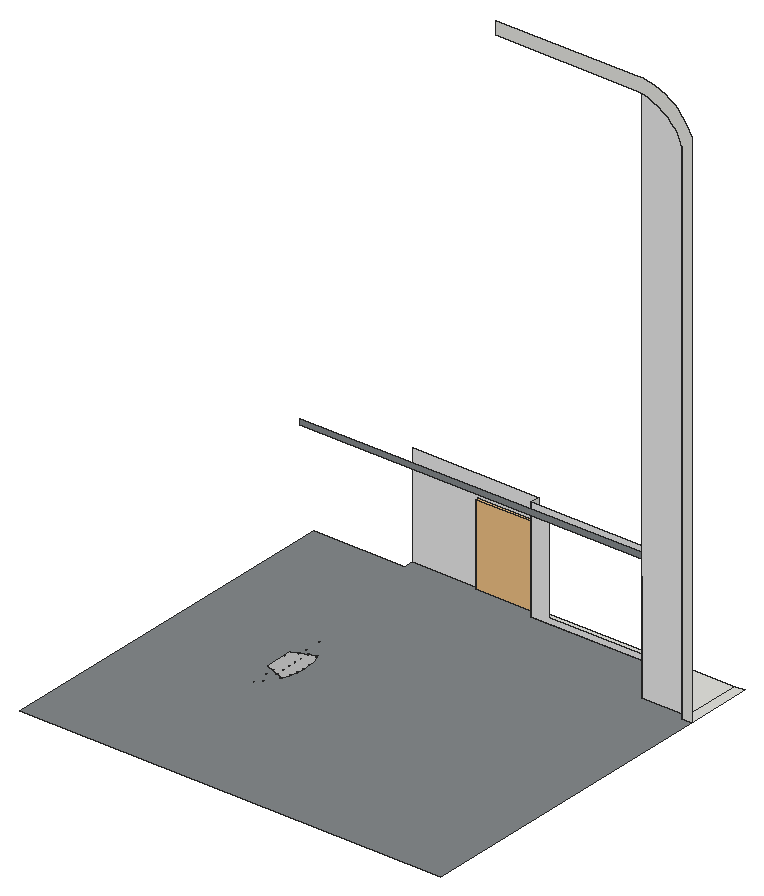
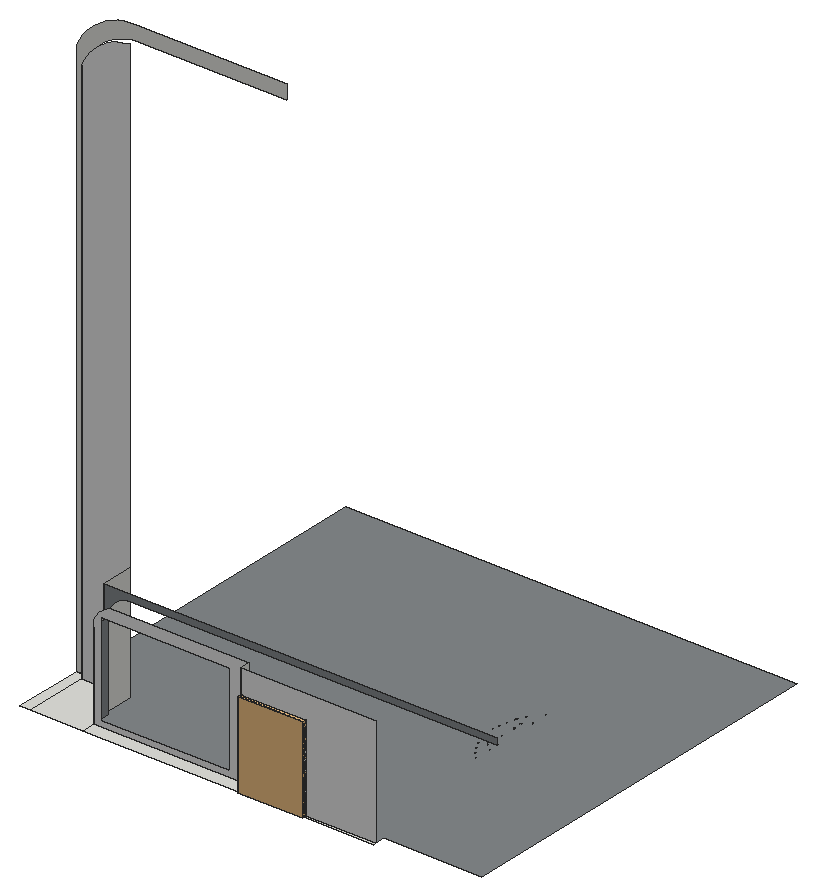
# SketchUp Ruby script. Lengths in inches.
U = 1.inch
M = Sketchup.active_model
def pt(a) = Geom::Point3d.new(a.map { |v| v * U })
def face(e, loops, mat)
  f = e.add_face(loops[0].map { |a| pt(a) })
  loops[1..].each { |l| e.add_face(l.map { |a| pt(a) }).erase! }
  f.material = f.back_material = mat if mat
  f
end
# faces: each face lists its corners as indices into pts; further lists are holes
def faces(e, pts, list, mat = nil) = list.each { |f| face(e, (f[0].is_a?(Array) ? f : [f]).map { |l| l.map { |i| pts[i] } }, mat) }
# xy, xz, yz: faces in a plane at the given z, y or x. An outline is a flat list of corners, or four numbers for a rectangle; further outlines are holes
def ring(l) = l.size == 4 ? [[l[0], l[1]], [l[2], l[1]], [l[2], l[3]], [l[0], l[3]]] : l.each_slice(2).to_a
def flat(e, list, mat, &to3) = list.each { |f| face(e, (f[0].is_a?(Array) ? f : [f]).map { |l| ring(l).map { |u, v| to3.(u, v) } }, mat) }
def xy(e, z, list, mat = nil) = flat(e, list, mat) { |x, y| [x, y, z] }
def xz(e, y, list, mat = nil) = flat(e, list, mat) { |x, z| [x, y, z] }
def yz(e, x, list, mat = nil) = flat(e, list, mat) { |y, z| [x, y, z] }
def lines(e, pts, list) = list.each { |a, b| e.add_line(pt(pts[a]), pt(pts[b])) }
# prism: a flat outline (further loops are holes) pulled along v
def prism(e, loops, v, mat = nil)
  f = face(e, loops, mat); d = Geom::Vector3d.new(v.map { |x| x * U })
  f.pushpull(f.normal.samedirection?(d) ? d.length : -d.length)
end
def box(e, o, s, mat = nil) = prism(e, [[o, [o[0] + s[0], o[1], o[2]], [o[0] + s[0], o[1] + s[1], o[2]], [o[0], o[1] + s[1], o[2]]]], [0, 0, s[2]], mat)
def at(x, y, z, deg = 0) = Geom::Transformation.translation(pt([x, y, z])) * Geom::Transformation.rotation(ORIGIN, Z_AXIS, deg.degrees)
def axes(o, x, y, z) = Geom::Transformation.new([*x, 0, *y, 0, *z, 0, *pt(o).to_a, 1])
def part(name) = M.definitions.add(name)
# library, detail: a bought-in or finely detailed component or shape, given as its bounding box
def library(name, o, s) = part(name).tap { |d| box(d.entities, o, s) }
def detail(e, o, s) = box(e.add_group.entities, o, s)
def put(e, d, t, mat = nil) = e.add_instance(d, t).tap { |i| i.material = mat if mat }
def group(e, t, mat = nil) = e.add_group.tap { |g| g.transformation = t; g.material = mat if mat }.entities
root = M.entities
M.materials.add("[Blacktop Old 01]").color = [132, 136, 139]
M.materials.add("[Metal_Steel_Textured_White]").color = [191, 191, 191]
M.materials.add("[Polished Concrete Old]").color = [229, 229, 229]
c1 = library("Glazed door",[-33.63,86.05,37.23],[27.33,3.12,36.46])
xy(root,3.625,[[303.95,218.965,308.325,249.09],[283.369,221.902,303.95,221.902,303.95,249.09,281.798,249.09,281.798,235.715,283.369,235.715],[215.602,243.402,281.798,249.09],[158.149,247.965,187.79,249.09]])
xy(root,3.625,[[116.615,76.29,308.325,76.29,308.325,218.965,303.95,218.965,303.95,221.902,283.369,221.902,283.369,235.715,281.798,235.715,281.798,243.402,215.602,243.402,215.602,249.09,187.79,249.09,187.79,247.965,158.149,247.965,158.149,243.402,116.615,243.402]],"[Blacktop Old 01]")
xy(root,3.625,[[[168.355,144.804,168.345,144.805,168.337,144.809,168.329,144.815,168.323,144.822,168.32,144.831,168.318,144.84,168.32,144.85,168.323,144.859,168.329,144.866,168.337,144.872,168.345,144.876,168.355,144.877,168.364,144.876,168.373,144.872,168.381,144.866,168.387,144.859,168.39,144.85,168.392,144.84,168.39,144.831,168.387,144.822,168.381,144.815,168.373,144.809,168.364,144.805],[168.355,144.82,168.36,144.821,168.365,144.823,168.369,144.826,168.372,144.83,168.374,144.835,168.375,144.84,168.374,144.846,168.372,144.85,168.369,144.854,168.365,144.858,168.36,144.86,168.35,144.86,168.345,144.858,168.341,144.854,168.338,144.85,168.336,144.846,168.335,144.84,168.336,144.835,168.338,144.83,168.341,144.826,168.345,144.823,168.35,144.821]],[168.355,144.82,168.35,144.821,168.345,144.823,168.341,144.826,168.338,144.83,168.336,144.835,168.335,144.84,168.336,144.846,168.338,144.85,168.341,144.854,168.345,144.858,168.35,144.86,168.36,144.86,168.365,144.858,168.369,144.854,168.372,144.85,168.374,144.846,168.375,144.84,168.374,144.835,168.372,144.83,168.369,144.826,168.365,144.823,168.36,144.821],[[170.535,147.224,170.512,147.227,170.49,147.236,170.472,147.25,170.458,147.269,170.449,147.29,170.446,147.313,170.449,147.336,170.458,147.358,170.472,147.376,170.49,147.39,170.512,147.399,170.535,147.402,170.558,147.399,170.579,147.39,170.597,147.376,170.612,147.358,170.62,147.336,170.624,147.313,170.62,147.29,170.612,147.269,170.597,147.25,170.579,147.236,170.558,147.227],[170.535,147.225,170.557,147.228,170.579,147.237,170.597,147.251,170.611,147.269,170.62,147.29,170.623,147.313,170.62,147.336,170.611,147.357,170.597,147.375,170.579,147.389,170.557,147.398,170.535,147.401,170.512,147.398,170.491,147.389,170.472,147.375,170.458,147.357,170.45,147.336,170.447,147.313,170.45,147.29,170.458,147.269,170.472,147.251,170.491,147.237,170.512,147.228]],[[172.387,149.952,172.364,149.955,172.343,149.964,172.325,149.978,172.311,149.996,172.302,150.017,172.299,150.04,172.302,150.0625,172.311,150.084,172.325,150.102,172.343,150.116,172.364,150.125,172.387,150.128,172.41,150.125,172.431,150.116,172.449,150.102,172.463,150.084,172.472,150.0625,172.475,150.04,172.472,150.017,172.463,149.996,172.449,149.978,172.431,149.964,172.41,149.955],[172.387,150.003,172.396,150.005,172.405,150.008,172.413,150.014,172.418,150.022,172.422,150.03,172.423,150.04,172.422,150.049,172.418,150.058,172.413,150.066,172.405,150.072,172.396,150.075,172.387,150.077,172.377,150.075,172.368,150.072,172.361,150.066,172.355,150.058,172.351,150.049,172.35,150.04,172.351,150.03,172.355,150.022,172.361,150.014,172.368,150.008,172.377,150.005]],[[168.197,151.934,168.174,151.937,168.153,151.946,168.135,151.96,168.121,151.978,168.112,151.999,168.109,152.022,168.112,152.045,168.121,152.066,168.135,152.084,168.153,152.098,168.174,152.107,168.197,152.11,168.22,152.107,168.241,152.098,168.259,152.084,168.273,152.066,168.282,152.045,168.285,152.022,168.282,151.999,168.273,151.978,168.259,151.96,168.241,151.946,168.22,151.937],[168.197,151.985,168.206,151.986,168.215,151.99,168.223,151.996,168.228,152.003,168.232,152.012,168.233,152.022,168.232,152.031,168.228,152.04,168.223,152.048,168.215,152.053,168.206,152.057,168.197,152.058,168.187,152.057,168.178,152.053,168.171,152.048,168.165,152.04,168.161,152.031,168.16,152.022,168.161,152.012,168.165,152.003,168.171,151.996,168.178,151.99,168.187,151.986]],
  [168.192,152.002,168.187,152.004,168.179,152.012,168.177,152.017,168.177,152.027,168.179,152.032,168.183,152.036,168.187,152.039,168.192,152.041,168.197,152.042,168.202,152.041,168.207,152.039,168.211,152.036,168.214,152.032,168.216,152.027,168.217,152.022,168.216,152.017,168.214,152.012,168.211,152.008,168.207,152.004,168.202,152.002],[[173.882,152.889,173.859,152.892,173.838,152.901,173.819,152.915,173.805,152.933,173.796,152.955,173.793,152.978,173.796,153.001,173.805,153.022,173.819,153.04,173.838,153.055,173.859,153.063,173.882,153.066,173.905,153.063,173.927,153.055,173.945,153.04,173.959,153.022,173.968,153.001,173.971,152.978,173.968,152.955,173.959,152.933,173.945,152.915,173.927,152.901,173.905,152.892],[173.882,152.89,173.905,152.893,173.926,152.901,173.944,152.915,173.958,152.934,173.967,152.955,173.97,152.978,173.967,153,173.958,153.022,173.944,153.04,173.926,153.054,173.905,153.0625,173.882,153.066,173.859,153.0625,173.838,153.054,173.82,153.04,173.806,153.022,173.797,153,173.794,152.978,173.797,152.955,173.806,152.934,173.82,152.915,173.838,152.901,173.859,152.893]],[[173.882,152.941,173.873,152.942,173.864,152.946,173.856,152.952,173.85,152.959,173.847,152.968,173.846,152.978,173.847,152.987,173.85,152.996,173.856,153.003,173.864,153.009,173.873,153.013,173.882,153.014,173.892,153.013,173.9,153.009,173.908,153.003,173.914,152.996,173.917,152.987,173.919,152.978,173.917,152.968,173.914,152.959,173.908,152.952,173.9,152.946,173.892,152.942],[173.877,152.958,173.887,152.958,173.892,152.96,173.896,152.963,173.899,152.968,173.901,152.972,173.902,152.978,173.901,152.983,173.899,152.988,173.896,152.992,173.892,152.995,173.887,152.997,173.882,152.998,173.877,152.997,173.872,152.995,173.868,152.992,173.865,152.988,173.863,152.983,173.862,152.978,173.863,152.972,173.865,152.968,173.868,152.963,173.872,152.96]],[173.877,152.958,173.872,152.96,173.868,152.963,173.865,152.968,173.863,152.972,173.862,152.978,173.863,152.983,173.865,152.988,173.868,152.992,173.872,152.995,173.877,152.997,173.882,152.998,173.887,152.997,173.892,152.995,173.896,152.992,173.899,152.988,173.901,152.983,173.902,152.978,173.901,152.972,173.899,152.968,173.896,152.963,173.892,152.96,173.887,152.958],[[174.407,153.192,164.789,157.176,164.789,169.578,174.407,173.5625,175.02,171.932,175.526,170.266,175.921,168.57,176.205,166.851,176.375,165.118,176.432,163.377,176.375,161.637,176.205,159.904,175.921,158.185,175.526,156.489,175.02,154.822],[175.826,166.578,175.849,166.581,175.87,166.59,175.889,166.604,175.903,166.623,175.912,166.644,175.915,166.667,175.912,166.69,175.903,166.712,175.889,166.73,175.87,166.744,175.849,166.753,175.826,166.756,175.803,166.753,175.782,166.744,175.763,166.73,175.749,166.712,175.74,166.69,175.737,166.667,175.74,166.644,175.749,166.623,175.763,166.604,175.782,166.59,175.803,166.581],[174.1875,172.951,174.211,172.954,174.232,172.963,174.251,172.977,174.265,172.995,174.274,173.017,174.277,173.04,174.274,173.0625,174.265,173.084,174.251,173.102,174.232,173.117,174.211,173.125,174.1875,173.128,174.165,173.125,174.143,173.117,174.125,173.102,174.111,173.084,174.102,173.0625,174.099,173.04,174.102,173.017,174.111,172.995,174.125,172.977,174.143,172.963,174.165,172.954],[175.208,156.761,175.231,156.764,175.252,156.773,175.27,156.787,175.285,156.805,175.293,156.827,175.296,156.85,175.293,156.873,175.285,156.894,175.27,156.913,175.252,156.927,175.231,156.936,175.208,156.939,175.185,156.936,175.163,156.927,175.145,156.913,175.131,156.894,175.122,156.873,175.119,156.85,175.122,156.827,175.131,156.805,175.145,156.787,175.163,156.773,175.185,156.764],[170.843,161.633,170.866,161.636,170.888,161.645,170.906,161.659,170.92,161.678,170.929,161.699,170.932,161.722,170.929,161.745,170.92,161.766,170.906,161.785,170.888,161.799,170.866,161.808,170.843,161.811,170.82,161.808,170.799,161.799,170.781,161.785,170.766,161.766,170.758,161.745,170.754,161.722,170.758,161.699,170.766,161.678,170.781,161.659,170.799,161.645,170.82,161.636],[165.188,169.223,165.211,169.226,165.232,169.235,165.251,169.249,165.265,169.267,165.274,169.289,165.277,169.312,165.274,169.335,165.265,169.356,165.251,169.375,165.232,169.389,165.211,169.398,165.188,169.401,165.165,169.398,165.143,169.389,165.125,169.375,165.111,169.356,165.102,169.335,165.099,169.312,165.102,169.289,165.111,169.267,165.125,169.249,165.143,169.235,165.165,169.226],[175.826,159.999,175.849,160.002,175.87,160.011,175.889,160.025,175.903,160.043,175.912,160.065,175.915,160.088,175.912,160.111,175.903,160.132,175.889,160.15,175.87,160.165,175.849,160.173,175.826,160.177,175.803,160.173,175.782,160.165,175.763,160.15,175.749,160.132,175.74,160.111,175.737,160.088,175.74,160.065,175.749,160.043,175.763,160.025,175.782,160.011,175.803,160.002],[168.188,156.112,168.211,156.115,168.232,156.124,168.251,156.138,168.265,156.156,168.274,156.177,168.277,156.2,168.274,156.223,168.265,156.245,168.251,156.263,168.232,156.277,168.211,156.286,168.188,156.289,168.165,156.286,168.143,156.277,168.125,156.263,168.111,156.245,168.102,156.223,168.099,156.2,168.102,156.177,168.111,156.156,168.125,156.138,168.143,156.124,168.165,156.115],[175.208,169.816,175.231,169.819,175.252,169.828,175.27,169.842,175.285,169.861,175.293,169.882,175.296,169.905,175.293,169.928,175.285,169.949,175.27,169.968,175.252,169.982,175.231,169.991,175.208,169.994,175.185,169.991,175.163,169.982,175.145,169.968,175.131,169.949,175.122,169.928,175.119,169.905,175.122,169.882,175.131,169.861,175.145,169.842,175.163,169.828,175.185,169.819],[165.188,160.321,165.211,160.324,165.232,160.333,165.251,160.347,165.265,160.366,165.274,160.387,165.277,160.41,165.274,160.433,165.265,160.455,165.251,160.473,165.232,160.487,165.211,160.496,165.188,160.499,165.165,160.496,165.143,160.487,165.125,160.473,165.111,160.455,165.102,160.433,165.099,160.41,165.102,160.387,165.111,160.366,165.125,160.347,165.143,160.333,165.165,160.324],[165.188,163.289,165.211,163.292,165.232,163.3,165.251,163.315,165.265,163.333,165.274,163.354,165.277,163.377,165.274,163.4,165.265,163.422,165.251,163.44,165.232,163.454,165.211,163.463,165.188,163.466,165.165,163.463,165.143,163.454,165.125,163.44,165.111,163.422,165.102,163.4,165.099,163.377,165.102,163.354,165.111,163.333,165.125,163.315,165.143,163.3,165.165,163.292],[170.843,158.322,170.866,158.325,170.888,158.334,170.906,158.348,170.92,158.367,170.929,158.388,170.932,158.411,170.929,158.434,170.92,158.456,170.906,158.474,170.888,158.488,170.866,158.497,170.843,158.5,170.82,158.497,170.799,158.488,170.781,158.474,170.766,158.456,170.758,158.434,170.754,158.411,170.758,158.388,170.766,158.367,170.781,158.348,170.799,158.334,170.82,158.325],[165.188,166.256,165.211,166.259,165.232,166.268,165.251,166.282,165.265,166.3,165.274,166.322,165.277,166.345,165.274,166.368,165.265,166.389,165.251,166.407,165.232,166.422,165.211,166.43,165.188,166.433,165.165,166.43,165.143,166.422,165.125,166.407,165.111,166.389,165.102,166.368,165.099,166.345,165.102,166.322,165.111,166.3,165.125,166.282,165.143,166.268,165.165,166.259],[168.188,170.465,168.211,170.468,168.232,170.477,168.251,170.492,168.265,170.51,168.274,170.531,168.277,170.554,168.274,170.577,168.265,170.599,168.251,170.617,168.232,170.631,168.211,170.64,168.188,170.643,168.165,170.64,168.143,170.631,168.125,170.617,168.111,170.599,168.102,170.577,168.099,170.554,168.102,170.531,168.111,170.51,168.125,170.492,168.143,170.477,168.165,170.468],[174.1875,153.626,174.211,153.629,174.232,153.638,174.251,153.652,174.265,153.671,174.274,153.692,174.277,153.715,174.274,153.738,174.265,153.76,174.251,153.778,174.232,153.792,174.211,153.801,174.1875,153.804,174.165,153.801,174.143,153.792,174.125,153.778,174.111,153.76,174.102,153.738,174.099,153.715,174.102,153.692,174.111,153.671,174.125,153.652,174.143,153.638,174.165,153.629],[165.188,157.354,165.211,157.357,165.232,157.366,165.251,157.38,165.265,157.399,165.274,157.42,165.277,157.443,165.274,157.466,165.265,157.488,165.251,157.506,165.232,157.52,165.211,157.529,165.188,157.532,165.165,157.529,165.143,157.52,165.125,157.506,165.111,157.488,165.102,157.466,165.099,157.443,165.102,157.42,165.111,157.399,165.125,157.38,165.143,157.366,165.165,157.357],[171.188,154.869,171.211,154.872,171.232,154.881,171.251,154.895,171.265,154.913,171.274,154.935,171.277,154.958,171.274,154.981,171.265,155.002,171.251,155.021,171.232,155.035,171.211,155.044,171.188,155.047,171.165,155.044,171.143,155.035,171.125,155.021,171.111,155.002,171.102,154.981,171.099,154.958,171.102,154.935,171.111,154.913,171.125,154.895,171.143,154.881,171.165,154.872],[170.843,168.255,170.866,168.258,170.888,168.267,170.906,168.281,170.92,168.299,170.929,168.321,170.932,168.344,170.929,168.367,170.92,168.388,170.906,168.406,170.888,168.421,170.866,168.429,170.843,168.432,170.82,168.429,170.799,168.421,170.781,168.406,170.766,168.388,170.758,168.367,170.754,168.344,170.758,168.321,170.766,168.299,170.781,168.281,170.799,168.267,170.82,168.258],[171.188,171.708,171.211,171.711,171.232,171.72,171.251,171.734,171.265,171.753,171.274,171.774,171.277,171.797,171.274,171.82,171.265,171.841,171.251,171.86,171.232,171.874,171.211,171.883,171.188,171.886,171.165,171.883,171.143,171.874,171.125,171.86,171.111,171.841,171.102,171.82,171.099,171.797,171.102,171.774,171.111,171.753,171.125,171.734,171.143,171.72,171.165,171.711],[170.843,164.944,170.866,164.947,170.888,164.956,170.906,164.97,170.92,164.988,170.929,165.01,170.932,165.033,170.929,165.056,170.92,165.077,170.906,165.096,170.888,165.11,170.866,165.119,170.843,165.122,170.82,165.119,170.799,165.11,170.781,165.096,170.766,165.077,170.758,165.056,170.754,165.033,170.758,165.01,170.766,164.988,170.781,164.97,170.799,164.956,170.82,164.947],[176.033,163.289,176.056,163.292,176.078,163.3,176.096,163.315,176.11,163.333,176.119,163.354,176.122,163.377,176.119,163.4,176.11,163.422,176.096,163.44,176.078,163.454,176.056,163.463,176.033,163.466,176.01,163.463,175.989,163.454,175.97,163.44,175.956,163.422,175.947,163.4,175.944,163.377,175.947,163.354,175.956,163.333,175.97,163.315,175.989,163.3,176.01,163.292]],
  [174.1875,153.695,174.183,153.696,174.178,153.698,174.174,153.701,174.17,153.705,174.168,153.71,174.168,153.72,174.17,153.725,174.178,153.733,174.183,153.735,174.193,153.735,174.198,153.733,174.202,153.729,174.205,153.725,174.207,153.72,174.208,153.715,174.207,153.71,174.205,153.705,174.202,153.701,174.198,153.698,174.193,153.696],[[170.882,154.184,170.873,154.185,170.864,154.189,170.856,154.194,170.85,154.202,170.847,154.211,170.846,154.22,170.847,154.23,170.85,154.239,170.856,154.246,170.864,154.252,170.873,154.256,170.882,154.257,170.892,154.256,170.9,154.252,170.908,154.246,170.914,154.239,170.918,154.23,170.919,154.22,170.918,154.211,170.914,154.202,170.908,154.194,170.9,154.189,170.892,154.185],[170.882,154.2,170.887,154.201,170.892,154.203,170.896,154.206,170.899,154.21,170.901,154.215,170.902,154.22,170.901,154.225,170.899,154.23,170.896,154.234,170.892,154.237,170.887,154.239,170.882,154.24,170.877,154.239,170.872,154.237,170.868,154.234,170.865,154.23,170.863,154.225,170.862,154.22,170.863,154.215,170.865,154.21,170.868,154.206,170.872,154.203,170.877,154.201]],[170.882,154.2,170.877,154.201,170.872,154.203,170.868,154.206,170.865,154.21,170.863,154.215,170.862,154.22,170.863,154.225,170.865,154.23,170.868,154.234,170.872,154.237,170.877,154.239,170.882,154.24,170.887,154.239,170.892,154.237,170.896,154.234,170.899,154.23,170.901,154.225,170.902,154.22,170.901,154.215,170.899,154.21,170.896,154.206,170.892,154.203,170.887,154.201],[[171.188,154.921,171.178,154.923,171.169,154.926,171.162,154.932,171.156,154.94,171.152,154.948,171.151,154.958,171.152,154.967,171.156,154.976,171.162,154.984,171.169,154.99,171.178,154.993,171.188,154.994,171.197,154.993,171.206,154.99,171.214,154.984,171.219,154.976,171.223,154.967,171.224,154.958,171.223,154.948,171.219,154.94,171.214,154.932,171.206,154.926,171.197,154.923],[171.188,154.938,171.193,154.939,171.198,154.941,171.202,154.944,171.205,154.948,171.207,154.953,171.208,154.958,171.207,154.963,171.205,154.968,171.202,154.972,171.198,154.975,171.193,154.977,171.188,154.978,171.183,154.977,171.178,154.975,171.174,154.972,171.17,154.968,171.168,154.963,171.168,154.953,171.17,154.948,171.174,154.944,171.178,154.941,171.183,154.939]],[171.188,154.938,171.183,154.939,171.178,154.941,171.174,154.944,171.17,154.948,171.168,154.953,171.168,154.963,171.17,154.968,171.174,154.972,171.178,154.975,171.183,154.977,171.188,154.978,171.193,154.977,171.198,154.975,171.202,154.972,171.205,154.968,171.207,154.963,171.208,154.958,171.207,154.953,171.205,154.948,171.202,154.944,171.198,154.941,171.193,154.939],
  [[175.208,156.761,175.185,156.764,175.163,156.773,175.145,156.787,175.131,156.805,175.122,156.827,175.119,156.85,175.122,156.873,175.131,156.894,175.145,156.913,175.163,156.927,175.185,156.936,175.208,156.939,175.231,156.936,175.252,156.927,175.27,156.913,175.285,156.894,175.293,156.873,175.296,156.85,175.293,156.827,175.285,156.805,175.27,156.787,175.252,156.773,175.231,156.764],[175.208,156.762,175.23,156.765,175.252,156.774,175.27,156.788,175.284,156.806,175.292,156.827,175.295,156.85,175.292,156.873,175.284,156.894,175.27,156.912,175.252,156.926,175.23,156.935,175.208,156.938,175.185,156.935,175.164,156.926,175.145,156.912,175.131,156.894,175.123,156.873,175.12,156.85,175.123,156.827,175.131,156.806,175.145,156.788,175.164,156.774,175.185,156.765]],[[175.208,156.813,175.198,156.814,175.189,156.818,175.182,156.824,175.176,156.832,175.172,156.84,175.171,156.85,175.172,156.859,175.176,156.868,175.182,156.876,175.189,156.882,175.198,156.885,175.208,156.886,175.217,156.885,175.226,156.882,175.233,156.876,175.239,156.868,175.243,156.859,175.244,156.85,175.243,156.84,175.239,156.832,175.233,156.824,175.226,156.818,175.217,156.814],[175.208,156.83,175.213,156.831,175.218,156.833,175.222,156.836,175.225,156.84,175.227,156.845,175.227,156.855,175.225,156.86,175.222,156.864,175.218,156.867,175.213,156.869,175.208,156.87,175.202,156.869,175.198,156.867,175.193,156.864,175.19,156.86,175.188,156.855,175.1875,156.85,175.188,156.845,175.19,156.84,175.193,156.836,175.198,156.833,175.202,156.831]],[175.208,156.83,175.202,156.831,175.198,156.833,175.193,156.836,175.19,156.84,175.188,156.845,175.1875,156.85,175.188,156.855,175.19,156.86,175.193,156.864,175.198,156.867,175.202,156.869,175.208,156.87,175.213,156.869,175.218,156.867,175.222,156.864,175.225,156.86,175.227,156.855,175.227,156.845,175.225,156.84,175.222,156.836,175.218,156.833,175.213,156.831],[[170.843,158.322,170.82,158.325,170.799,158.334,170.781,158.348,170.766,158.367,170.758,158.388,170.754,158.411,170.758,158.434,170.766,158.456,170.781,158.474,170.799,158.488,170.82,158.497,170.843,158.5,170.866,158.497,170.888,158.488,170.906,158.474,170.92,158.456,170.929,158.434,170.932,158.411,170.929,158.388,170.92,158.367,170.906,158.348,170.888,158.334,170.866,158.325],[170.843,158.323,170.866,158.326,170.887,158.335,170.906,158.349,170.92,158.367,170.928,158.389,170.931,158.411,170.928,158.434,170.92,158.455,170.906,158.473,170.887,158.487,170.866,158.496,170.843,158.499,170.821,158.496,170.799,158.487,170.781,158.473,170.767,158.455,170.758,158.434,170.755,158.411,170.758,158.389,170.767,158.367,170.781,158.349,170.799,158.335,170.821,158.326]],[[170.843,158.323,170.821,158.326,170.799,158.335,170.781,158.349,170.767,158.367,170.758,158.389,170.755,158.411,170.758,158.434,170.767,158.455,170.781,158.473,170.799,158.487,170.821,158.496,170.843,158.499,170.866,158.496,170.887,158.487,170.906,158.473,170.92,158.455,170.928,158.434,170.931,158.411,170.928,158.389,170.92,158.367,170.906,158.349,170.887,158.335,170.866,158.326],[170.843,158.375,170.853,158.376,170.862,158.38,170.869,158.385,170.875,158.393,170.879,158.402,170.88,158.411,170.879,158.421,170.875,158.43,170.869,158.437,170.862,158.443,170.853,158.447,170.843,158.448,170.834,158.447,170.825,158.443,170.818,158.437,170.812,158.43,170.808,158.421,170.807,158.411,170.808,158.402,170.812,158.393,170.818,158.385,170.825,158.38,170.834,158.376]],
  [170.843,158.391,170.838,158.392,170.833,158.394,170.829,158.397,170.826,158.401,170.824,158.406,170.823,158.411,170.824,158.416,170.826,158.421,170.829,158.425,170.833,158.429,170.838,158.431,170.849,158.431,170.853,158.429,170.858,158.425,170.861,158.421,170.863,158.416,170.863,158.406,170.861,158.401,170.858,158.397,170.853,158.394,170.849,158.392],[[175.826,159.999,175.803,160.002,175.782,160.011,175.763,160.025,175.749,160.043,175.74,160.065,175.737,160.088,175.74,160.111,175.749,160.132,175.763,160.15,175.782,160.165,175.803,160.173,175.826,160.177,175.849,160.173,175.87,160.165,175.889,160.15,175.903,160.132,175.912,160.111,175.915,160.088,175.912,160.065,175.903,160.043,175.889,160.025,175.87,160.011,175.849,160.002],[175.826,160,175.849,160.003,175.87,160.011,175.888,160.025,175.902,160.044,175.911,160.065,175.914,160.088,175.911,160.11,175.902,160.132,175.888,160.15,175.87,160.164,175.849,160.173,175.826,160.176,175.803,160.173,175.782,160.164,175.764,160.15,175.75,160.132,175.741,160.11,175.738,160.088,175.741,160.065,175.75,160.044,175.764,160.025,175.782,160.011,175.803,160.003]],[[175.826,160.051,175.817,160.052,175.808,160.056,175.8,160.062,175.794,160.069,175.791,160.078,175.789,160.088,175.791,160.097,175.794,160.106,175.8,160.113,175.808,160.119,175.817,160.123,175.826,160.124,175.835,160.123,175.844,160.119,175.852,160.113,175.858,160.106,175.861,160.097,175.863,160.088,175.861,160.078,175.858,160.069,175.852,160.062,175.844,160.056,175.835,160.052],[175.821,160.068,175.831,160.068,175.836,160.07,175.84,160.074,175.843,160.078,175.845,160.082,175.846,160.088,175.845,160.093,175.843,160.098,175.84,160.102,175.836,160.105,175.831,160.107,175.826,160.108,175.821,160.107,175.816,160.105,175.812,160.102,175.809,160.098,175.807,160.093,175.806,160.088,175.807,160.082,175.809,160.078,175.812,160.074,175.816,160.07]],[175.821,160.068,175.816,160.07,175.812,160.074,175.809,160.078,175.807,160.082,175.806,160.088,175.807,160.093,175.809,160.098,175.812,160.102,175.816,160.105,175.821,160.107,175.826,160.108,175.831,160.107,175.836,160.105,175.84,160.102,175.843,160.098,175.845,160.093,175.846,160.088,175.845,160.082,175.843,160.078,175.84,160.074,175.836,160.07,175.831,160.068],[[170.843,161.633,170.82,161.636,170.799,161.645,170.781,161.659,170.766,161.678,170.758,161.699,170.754,161.722,170.758,161.745,170.766,161.766,170.781,161.785,170.799,161.799,170.82,161.808,170.843,161.811,170.866,161.808,170.888,161.799,170.906,161.785,170.92,161.766,170.929,161.745,170.932,161.722,170.929,161.699,170.92,161.678,170.906,161.659,170.888,161.645,170.866,161.636],[170.843,161.634,170.866,161.637,170.887,161.646,170.906,161.66,170.92,161.678,170.928,161.699,170.931,161.722,170.928,161.745,170.92,161.766,170.906,161.784,170.887,161.798,170.866,161.807,170.843,161.81,170.821,161.807,170.799,161.798,170.781,161.784,170.767,161.766,170.758,161.745,170.755,161.722,170.758,161.699,170.767,161.678,170.781,161.66,170.799,161.646,170.821,161.637]],
  [[170.843,161.634,170.821,161.637,170.799,161.646,170.781,161.66,170.767,161.678,170.758,161.699,170.755,161.722,170.758,161.745,170.767,161.766,170.781,161.784,170.799,161.798,170.821,161.807,170.843,161.81,170.866,161.807,170.887,161.798,170.906,161.784,170.92,161.766,170.928,161.745,170.931,161.722,170.928,161.699,170.92,161.678,170.906,161.66,170.887,161.646,170.866,161.637],[170.843,161.685,170.853,161.687,170.862,161.69,170.869,161.696,170.875,161.704,170.879,161.713,170.88,161.722,170.879,161.732,170.875,161.74,170.869,161.748,170.862,161.754,170.853,161.757,170.843,161.759,170.834,161.757,170.825,161.754,170.818,161.748,170.812,161.74,170.808,161.732,170.807,161.722,170.808,161.713,170.812,161.704,170.818,161.696,170.825,161.69,170.834,161.687]],[175.944,163.377,175.947,163.4,175.956,163.422,175.97,163.44,175.989,163.454,176.01,163.463,176.033,163.466,176.056,163.463,176.078,163.454,176.096,163.44,176.11,163.422,176.119,163.4,176.122,163.377,176.121,163.377,176.118,163.4,176.109,163.421,176.095,163.44,176.077,163.454,176.056,163.462,176.033,163.465,176.01,163.462,175.989,163.454,175.971,163.44,175.957,163.421,175.948,163.4,175.945,163.377],[[170.843,164.944,170.82,164.947,170.799,164.956,170.781,164.97,170.766,164.988,170.758,165.01,170.754,165.033,170.758,165.056,170.766,165.077,170.781,165.096,170.799,165.11,170.82,165.119,170.843,165.122,170.866,165.119,170.888,165.11,170.906,165.096,170.92,165.077,170.929,165.056,170.932,165.033,170.929,165.01,170.92,164.988,170.906,164.97,170.888,164.956,170.866,164.947],[170.843,164.945,170.866,164.948,170.887,164.957,170.906,164.971,170.92,164.989,170.928,165.01,170.931,165.033,170.928,165.056,170.92,165.077,170.906,165.095,170.887,165.109,170.866,165.118,170.843,165.121,170.821,165.118,170.799,165.109,170.781,165.095,170.767,165.077,170.758,165.056,170.755,165.033,170.758,165.01,170.767,164.989,170.781,164.971,170.799,164.957,170.821,164.948]],[170.843,165.013,170.838,165.014,170.833,165.016,170.829,165.019,170.826,165.023,170.824,165.028,170.823,165.033,170.824,165.038,170.826,165.043,170.829,165.047,170.833,165.05,170.838,165.052,170.843,165.053,170.849,165.052,170.853,165.05,170.858,165.047,170.861,165.043,170.863,165.038,170.863,165.028,170.861,165.023,170.858,165.019,170.853,165.016,170.849,165.014],[[170.843,168.255,170.82,168.258,170.799,168.267,170.781,168.281,170.766,168.299,170.758,168.321,170.754,168.344,170.758,168.367,170.766,168.388,170.781,168.406,170.799,168.421,170.82,168.429,170.843,168.432,170.866,168.429,170.888,168.421,170.906,168.406,170.92,168.388,170.929,168.367,170.932,168.344,170.929,168.321,170.92,168.299,170.906,168.281,170.888,168.267,170.866,168.258],[170.843,168.256,170.866,168.259,170.887,168.267,170.906,168.281,170.92,168.3,170.928,168.321,170.931,168.344,170.928,168.366,170.92,168.388,170.906,168.406,170.887,168.42,170.866,168.429,170.843,168.432,170.821,168.429,170.799,168.42,170.781,168.406,170.767,168.388,170.758,168.366,170.755,168.344,170.758,168.321,170.767,168.3,170.781,168.281,170.799,168.267,170.821,168.259]],
  [[170.843,168.256,170.821,168.259,170.799,168.267,170.781,168.281,170.767,168.3,170.758,168.321,170.755,168.344,170.758,168.366,170.767,168.388,170.781,168.406,170.799,168.42,170.821,168.429,170.843,168.432,170.866,168.429,170.887,168.42,170.906,168.406,170.92,168.388,170.928,168.366,170.931,168.344,170.928,168.321,170.92,168.3,170.906,168.281,170.887,168.267,170.866,168.259],[170.843,168.307,170.853,168.308,170.862,168.312,170.869,168.318,170.875,168.325,170.879,168.334,170.88,168.344,170.879,168.353,170.875,168.362,170.869,168.369,170.862,168.375,170.853,168.379,170.843,168.38,170.834,168.379,170.825,168.375,170.818,168.369,170.812,168.362,170.808,168.353,170.807,168.344,170.808,168.334,170.812,168.325,170.818,168.318,170.825,168.312,170.834,168.308]],[[168.188,170.465,168.165,170.468,168.143,170.477,168.125,170.492,168.111,170.51,168.102,170.531,168.099,170.554,168.102,170.577,168.111,170.599,168.125,170.617,168.143,170.631,168.165,170.64,168.188,170.643,168.211,170.64,168.232,170.631,168.251,170.617,168.265,170.599,168.274,170.577,168.277,170.554,168.274,170.531,168.265,170.51,168.251,170.492,168.232,170.477,168.211,170.468],[168.188,170.466,168.211,170.469,168.232,170.478,168.25,170.492,168.264,170.51,168.273,170.532,168.276,170.554,168.273,170.577,168.264,170.598,168.25,170.617,168.232,170.631,168.211,170.639,168.188,170.642,168.165,170.639,168.144,170.631,168.126,170.617,168.112,170.598,168.103,170.577,168.1,170.554,168.103,170.532,168.112,170.51,168.126,170.492,168.144,170.478,168.165,170.469]],[[168.188,170.518,168.178,170.519,168.169,170.523,168.162,170.528,168.156,170.536,168.152,170.545,168.151,170.554,168.152,170.564,168.156,170.573,168.162,170.58,168.169,170.586,168.178,170.59,168.188,170.591,168.197,170.59,168.206,170.586,168.214,170.58,168.219,170.573,168.223,170.564,168.224,170.554,168.223,170.545,168.219,170.536,168.214,170.528,168.206,170.523,168.197,170.519],[168.188,170.534,168.193,170.535,168.198,170.537,168.202,170.54,168.205,170.544,168.207,170.549,168.208,170.554,168.207,170.56,168.205,170.564,168.202,170.568,168.198,170.572,168.193,170.574,168.183,170.574,168.178,170.572,168.17,170.564,168.168,170.56,168.168,170.549,168.17,170.544,168.174,170.54,168.178,170.537,168.183,170.535]],[168.188,170.534,168.183,170.535,168.178,170.537,168.174,170.54,168.17,170.544,168.168,170.549,168.168,170.56,168.17,170.564,168.178,170.572,168.183,170.574,168.193,170.574,168.198,170.572,168.202,170.568,168.205,170.564,168.207,170.56,168.208,170.554,168.207,170.549,168.205,170.544,168.202,170.54,168.198,170.537,168.193,170.535],[[167.882,171.203,167.859,171.206,167.838,171.215,167.819,171.229,167.805,171.248,167.796,171.269,167.793,171.292,167.796,171.315,167.805,171.336,167.819,171.355,167.838,171.369,167.859,171.378,167.882,171.381,167.905,171.378,167.927,171.369,167.945,171.355,167.959,171.336,167.968,171.315,167.971,171.292,167.968,171.269,167.959,171.248,167.945,171.229,167.927,171.215,167.905,171.206],[167.882,171.204,167.905,171.207,167.926,171.216,167.944,171.23,167.958,171.248,167.967,171.269,167.97,171.292,167.967,171.315,167.958,171.336,167.944,171.354,167.926,171.368,167.905,171.377,167.882,171.38,167.859,171.377,167.838,171.368,167.82,171.354,167.806,171.336,167.797,171.315,167.794,171.292,167.797,171.269,167.806,171.248,167.82,171.23,167.838,171.216,167.859,171.207]],
  [[171.188,171.709,171.165,171.712,171.144,171.721,171.126,171.735,171.112,171.753,171.103,171.774,171.1,171.797,171.103,171.82,171.112,171.841,171.126,171.859,171.144,171.873,171.165,171.882,171.188,171.885,171.21,171.882,171.232,171.873,171.25,171.859,171.264,171.841,171.273,171.82,171.276,171.797,171.273,171.774,171.264,171.753,171.25,171.735,171.232,171.721,171.21,171.712],[171.188,171.76,171.197,171.762,171.206,171.765,171.214,171.771,171.219,171.779,171.223,171.788,171.224,171.797,171.223,171.806,171.219,171.815,171.214,171.823,171.206,171.829,171.197,171.832,171.188,171.834,171.178,171.832,171.169,171.829,171.162,171.823,171.156,171.815,171.152,171.806,171.151,171.797,171.152,171.788,171.156,171.779,171.162,171.771,171.169,171.765,171.178,171.762]],[[170.882,172.498,170.873,172.499,170.864,172.503,170.856,172.509,170.85,172.516,170.847,172.525,170.846,172.535,170.847,172.544,170.85,172.553,170.856,172.561,170.864,172.566,170.873,172.57,170.882,172.571,170.892,172.57,170.9,172.566,170.908,172.561,170.914,172.553,170.918,172.544,170.919,172.535,170.918,172.525,170.914,172.516,170.908,172.509,170.9,172.503,170.892,172.499],[170.877,172.515,170.887,172.515,170.892,172.517,170.896,172.521,170.899,172.525,170.901,172.529,170.902,172.535,170.901,172.54,170.899,172.545,170.896,172.549,170.892,172.552,170.887,172.554,170.882,172.555,170.877,172.554,170.872,172.552,170.868,172.549,170.865,172.545,170.863,172.54,170.862,172.535,170.863,172.529,170.865,172.525,170.868,172.521,170.872,172.517]],[170.877,172.515,170.872,172.517,170.868,172.521,170.865,172.525,170.863,172.529,170.862,172.535,170.863,172.54,170.865,172.545,170.868,172.549,170.872,172.552,170.877,172.554,170.882,172.555,170.887,172.554,170.892,172.552,170.896,172.549,170.899,172.545,170.901,172.54,170.902,172.535,170.901,172.529,170.899,172.525,170.896,172.521,170.892,172.517,170.887,172.515],[[174.1875,172.951,174.165,172.954,174.143,172.963,174.125,172.977,174.111,172.995,174.102,173.017,174.099,173.04,174.102,173.0625,174.111,173.084,174.125,173.102,174.143,173.117,174.165,173.125,174.1875,173.128,174.211,173.125,174.232,173.117,174.251,173.102,174.265,173.084,174.274,173.0625,174.277,173.04,174.274,173.017,174.265,172.995,174.251,172.977,174.232,172.963,174.211,172.954],[174.1875,172.952,174.21,172.955,174.232,172.963,174.25,172.977,174.264,172.996,174.273,173.017,174.276,173.04,174.273,173.0625,174.264,173.084,174.25,173.102,174.232,173.116,174.21,173.125,174.1875,173.128,174.165,173.125,174.144,173.116,174.125,173.102,174.112,173.084,174.103,173.0625,174.1,173.04,174.103,173.017,174.112,172.996,174.125,172.977,174.144,172.963,174.165,172.955]],[[173.882,173.688,173.859,173.691,173.838,173.7,173.819,173.714,173.805,173.733,173.796,173.754,173.793,173.777,173.796,173.8,173.805,173.822,173.819,173.84,173.838,173.854,173.859,173.863,173.882,173.866,173.905,173.863,173.927,173.854,173.945,173.84,173.959,173.822,173.968,173.8,173.971,173.777,173.968,173.754,173.959,173.733,173.945,173.714,173.927,173.7,173.905,173.691],[173.882,173.689,173.905,173.692,173.926,173.701,173.944,173.715,173.958,173.733,173.967,173.755,173.97,173.777,173.967,173.8,173.958,173.821,173.944,173.839,173.926,173.853,173.905,173.862,173.882,173.865,173.859,173.862,173.838,173.853,173.82,173.839,173.806,173.821,173.797,173.8,173.794,173.777,173.797,173.755,173.806,173.733,173.82,173.715,173.838,173.701,173.859,173.692]],
  [[168.197,174.696,168.187,174.698,168.178,174.701,168.171,174.707,168.165,174.715,168.161,174.724,168.16,174.733,168.161,174.743,168.165,174.751,168.171,174.759,168.178,174.765,168.187,174.768,168.197,174.77,168.206,174.768,168.215,174.765,168.223,174.759,168.228,174.751,168.232,174.743,168.233,174.733,168.232,174.724,168.228,174.715,168.223,174.707,168.215,174.701,168.206,174.698],[168.197,174.713,168.202,174.714,168.207,174.716,168.211,174.719,168.214,174.723,168.216,174.728,168.217,174.733,168.216,174.738,168.214,174.743,168.211,174.747,168.207,174.75,168.202,174.752,168.197,174.753,168.192,174.752,168.187,174.75,168.183,174.747,168.179,174.743,168.177,174.738,168.177,174.728,168.179,174.723,168.183,174.719,168.187,174.716,168.192,174.714]],[168.197,174.713,168.192,174.714,168.187,174.716,168.183,174.719,168.179,174.723,168.177,174.728,168.177,174.738,168.179,174.743,168.183,174.747,168.187,174.75,168.192,174.752,168.197,174.753,168.202,174.752,168.207,174.75,168.211,174.747,168.214,174.743,168.216,174.738,168.217,174.733,168.216,174.728,168.214,174.723,168.211,174.719,168.207,174.716,168.202,174.714],[[172.387,176.626,172.364,176.629,172.342,176.638,172.324,176.652,172.31,176.67,172.301,176.692,172.298,176.715,172.301,176.738,172.31,176.759,172.324,176.778,172.342,176.792,172.364,176.801,172.387,176.804,172.41,176.801,172.431,176.792,172.45,176.778,172.464,176.759,172.473,176.738,172.476,176.715,172.473,176.692,172.464,176.67,172.45,176.652,172.431,176.638,172.41,176.629],[172.387,176.627,172.41,176.63,172.431,176.639,172.449,176.653,172.463,176.671,172.472,176.692,172.475,176.715,172.472,176.738,172.463,176.759,172.449,176.777,172.431,176.791,172.41,176.8,172.387,176.803,172.364,176.8,172.343,176.791,172.325,176.777,172.311,176.759,172.302,176.738,172.299,176.715,172.302,176.692,172.311,176.671,172.325,176.653,172.343,176.639,172.364,176.63]],[[172.387,176.627,172.364,176.63,172.343,176.639,172.325,176.653,172.311,176.671,172.302,176.692,172.299,176.715,172.302,176.738,172.311,176.759,172.325,176.777,172.343,176.791,172.364,176.8,172.387,176.803,172.41,176.8,172.431,176.791,172.449,176.777,172.463,176.759,172.472,176.738,172.475,176.715,172.472,176.692,172.463,176.671,172.449,176.653,172.431,176.639,172.41,176.63],[172.387,176.678,172.396,176.68,172.405,176.683,172.413,176.689,172.418,176.697,172.422,176.705,172.423,176.715,172.422,176.724,172.418,176.733,172.413,176.741,172.405,176.747,172.396,176.75,172.387,176.752,172.377,176.75,172.368,176.747,172.361,176.741,172.355,176.733,172.351,176.724,172.35,176.715,172.351,176.705,172.355,176.697,172.361,176.689,172.368,176.683,172.377,176.68]],[[170.535,179.353,170.512,179.356,170.49,179.365,170.472,179.379,170.458,179.397,170.449,179.419,170.446,179.442,170.449,179.465,170.458,179.486,170.472,179.505,170.49,179.519,170.512,179.528,170.535,179.531,170.558,179.528,170.579,179.519,170.597,179.505,170.612,179.486,170.62,179.465,170.624,179.442,170.62,179.419,170.612,179.397,170.597,179.379,170.579,179.365,170.558,179.356],[170.535,179.354,170.557,179.357,170.579,179.366,170.597,179.38,170.611,179.398,170.62,179.419,170.623,179.442,170.62,179.464,170.611,179.486,170.597,179.504,170.579,179.518,170.557,179.527,170.535,179.53,170.512,179.527,170.491,179.518,170.472,179.504,170.458,179.486,170.45,179.464,170.447,179.442,170.45,179.419,170.458,179.398,170.472,179.38,170.491,179.366,170.512,179.357]],
  [[170.535,179.405,170.525,179.406,170.516,179.41,170.509,179.416,170.503,179.423,170.499,179.432,170.498,179.442,170.499,179.451,170.503,179.46,170.509,179.468,170.516,179.473,170.525,179.477,170.535,179.478,170.544,179.477,170.553,179.473,170.561,179.468,170.566,179.46,170.57,179.451,170.571,179.442,170.57,179.432,170.566,179.423,170.561,179.416,170.553,179.41,170.544,179.406],[170.529,179.422,170.54,179.422,170.545,179.424,170.549,179.428,170.552,179.432,170.554,179.437,170.555,179.442,170.554,179.447,170.552,179.452,170.549,179.456,170.545,179.459,170.54,179.461,170.535,179.462,170.529,179.461,170.525,179.459,170.521,179.456,170.517,179.452,170.515,179.447,170.515,179.437,170.517,179.432,170.525,179.424]],[[168.355,181.826,168.332,181.829,168.31,181.837,168.292,181.852,168.278,181.87,168.269,181.891,168.266,181.914,168.269,181.9375,168.278,181.959,168.292,181.977,168.31,181.991,168.332,182,168.355,182.003,168.378,182,168.399,181.991,168.418,181.977,168.432,181.959,168.441,181.9375,168.444,181.914,168.441,181.891,168.432,181.87,168.418,181.852,168.399,181.837,168.378,181.829],[168.355,181.827,168.378,181.83,168.399,181.838,168.417,181.852,168.431,181.87,168.44,181.892,168.443,181.914,168.44,181.937,168.431,181.958,168.417,181.977,168.399,181.991,168.378,181.999,168.355,182.002,168.332,181.999,168.311,181.991,168.293,181.977,168.279,181.958,168.27,181.937,168.267,181.914,168.27,181.892,168.279,181.87,168.293,181.852,168.311,181.838,168.332,181.83]],[[168.355,181.878,168.345,181.879,168.337,181.883,168.329,181.889,168.323,181.896,168.32,181.905,168.318,181.914,168.32,181.924,168.323,181.933,168.329,181.94,168.337,181.946,168.345,181.95,168.355,181.951,168.364,181.95,168.373,181.946,168.381,181.94,168.387,181.933,168.39,181.924,168.392,181.914,168.39,181.905,168.387,181.896,168.381,181.889,168.373,181.883,168.364,181.879],[168.355,181.894,168.36,181.895,168.365,181.897,168.369,181.9,168.372,181.904,168.374,181.909,168.375,181.914,168.374,181.92,168.372,181.924,168.369,181.929,168.365,181.932,168.36,181.934,168.35,181.934,168.345,181.932,168.341,181.929,168.338,181.924,168.336,181.92,168.335,181.914,168.336,181.909,168.338,181.904,168.341,181.9,168.345,181.897,168.35,181.895]],[168.355,181.894,168.35,181.895,168.345,181.897,168.341,181.9,168.338,181.904,168.336,181.909,168.335,181.914,168.336,181.92,168.338,181.924,168.341,181.929,168.345,181.932,168.35,181.934,168.36,181.934,168.365,181.932,168.369,181.929,168.372,181.924,168.374,181.92,168.375,181.914,168.374,181.909,168.372,181.904,168.369,181.9,168.365,181.897,168.36,181.895]],"[Metal_Steel_Textured_White]")
xz(root,218.965,[[303.95,3.625,308.325,3.625,308.325,242.342,307.165,244.707,305.781,246.948,304.1875,249.045,303.95,249.302,302.398,250.978,300.492,252.674,300.43,252.729,298.302,254.281,296.034,255.619,293.646,256.732,291.163,257.609,288.606,258.241,286,258.622,283.369,258.75,219.138,258.75,219.138,252.674,283.369,252.674,283.369,252.57,284.398,252.49,286.735,252.074,289.02,251.432,291.232,250.569,293.348,249.494,295.348,248.216,297.214,246.749,298.927,245.106,300.472,243.304,301.832,241.358,302.995,239.289,303.95,237.116]])
xz(root,221.902,[[283.369,3.625,303.95,3.625,303.95,237.116,302.995,239.289,301.832,241.358,300.472,243.304,298.927,245.106,297.214,246.749,295.348,248.216,293.348,249.494,291.232,250.569,289.02,251.432,286.735,252.074,284.398,252.49,283.369,252.57]],"[Polished Concrete Old]")
xz(root,235.715,[[281.798,3.625,283.369,3.625,283.369,53.067,116.615,53.067,116.615,50.25,272.073,50.25,273.343,50.167,274.59,49.919,275.795,49.51,276.936,48.947,277.993,48.24,278.95,47.402,279.789,46.445,280.495,45.388,281.058,44.247,281.467,43.042,281.715,41.795,281.798,40.525]],"[Blacktop Old 01]")
xz(root,243.402,[[[215.602,3.625,281.798,3.625,281.798,40.525,281.715,41.795,281.467,43.042,281.058,44.247,280.495,45.388,279.789,46.445,278.95,47.402,277.993,48.24,276.936,48.947,275.795,49.51,274.59,49.919,273.343,50.167,272.073,50.25,215.602,50.25],[223.8,6.055,278.487,45.43]]],"[Polished Concrete Old]")
xz(root,247.965,[[158.149,3.625,187.79,3.625,187.79,40.089,215.602,40.089,215.602,50.25,158.149,50.25]],"[Polished Concrete Old]")
xz(root,249.09,[[187.79,3.625,215.602,40.089]])
yz(root,187.79,[[247.965,3.625,249.09,40.089]])
yz(root,215.602,[[243.402,3.625,243.402,50.25,247.965,50.25,247.965,40.089,249.09,40.089,249.09,3.625]])
yz(root,281.798,[[235.715,3.625,243.402,40.525]],"[Blacktop Old 01]")
yz(root,283.369,[[221.902,3.625,235.715,53.067]])
yz(root,303.95,[[218.965,3.625,221.902,237.116]])
put(root,c1,at(221.42,160.55,-33.6))
